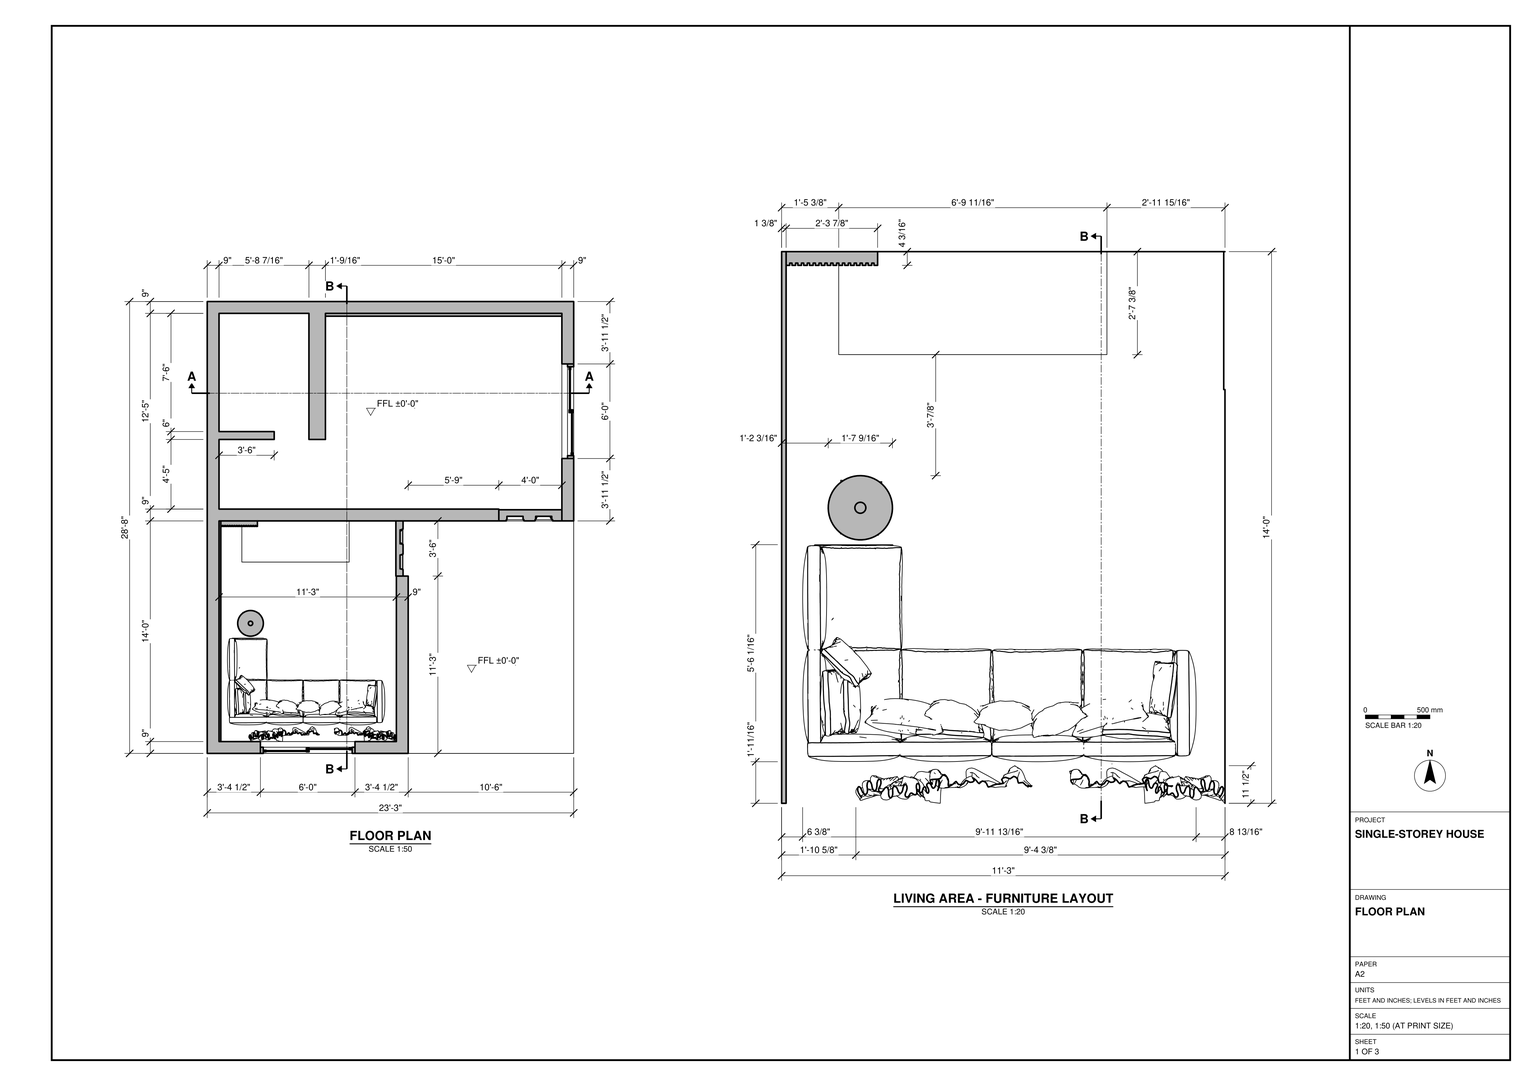
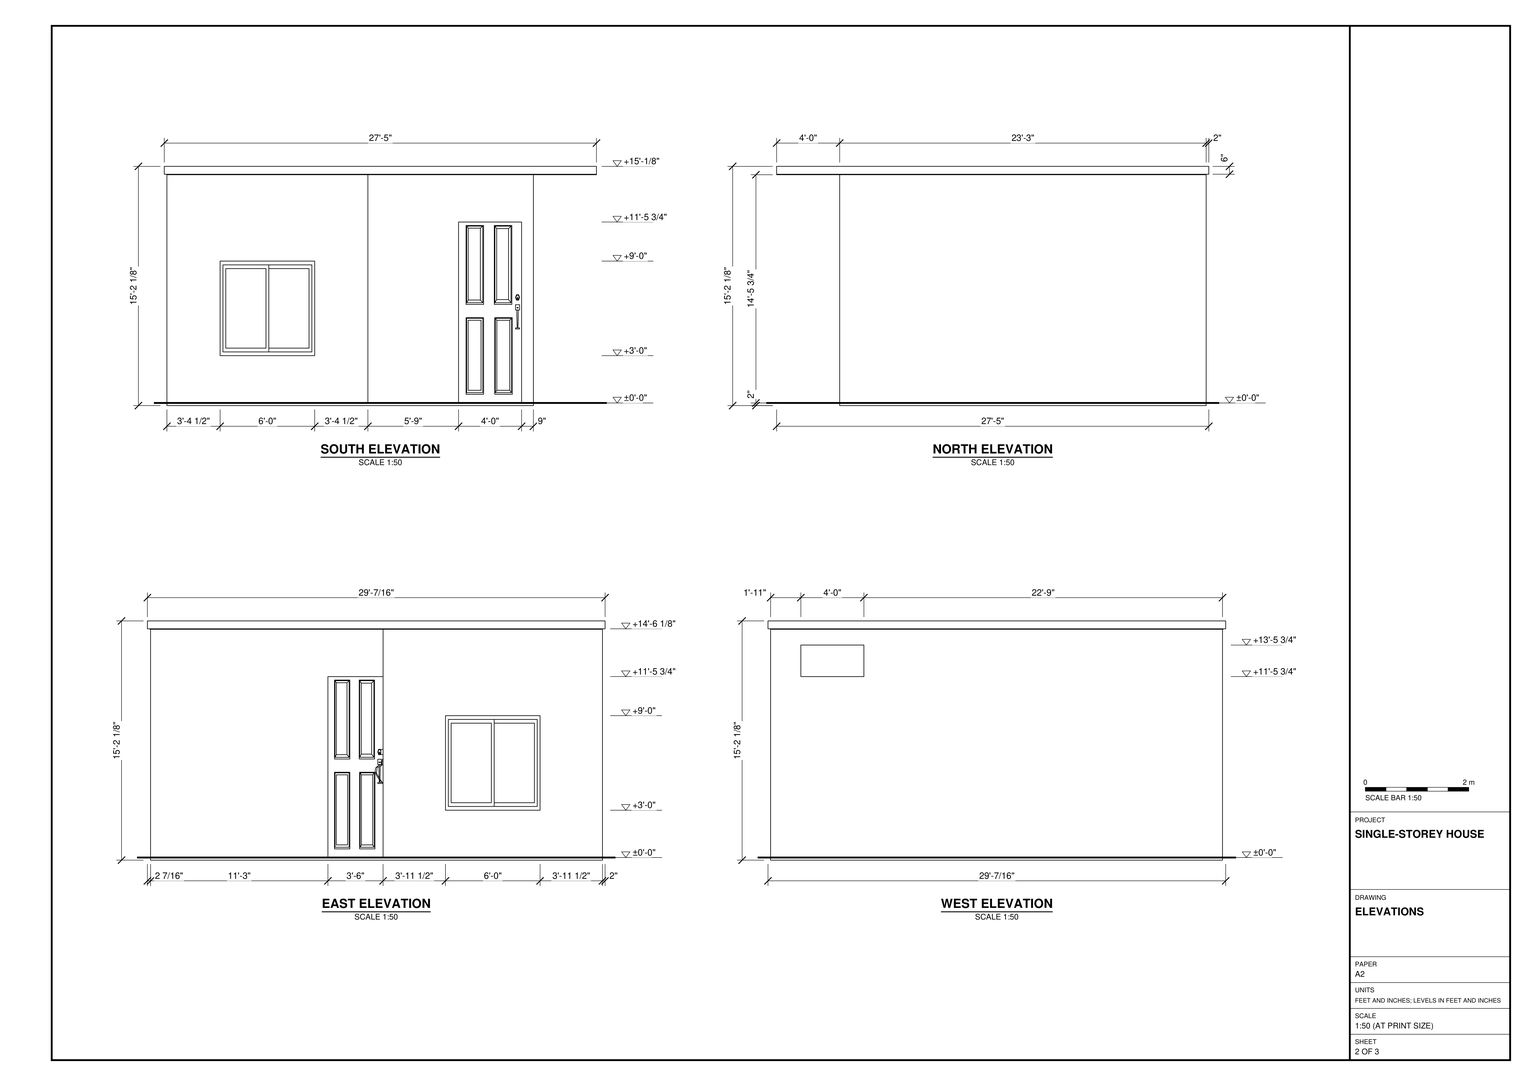
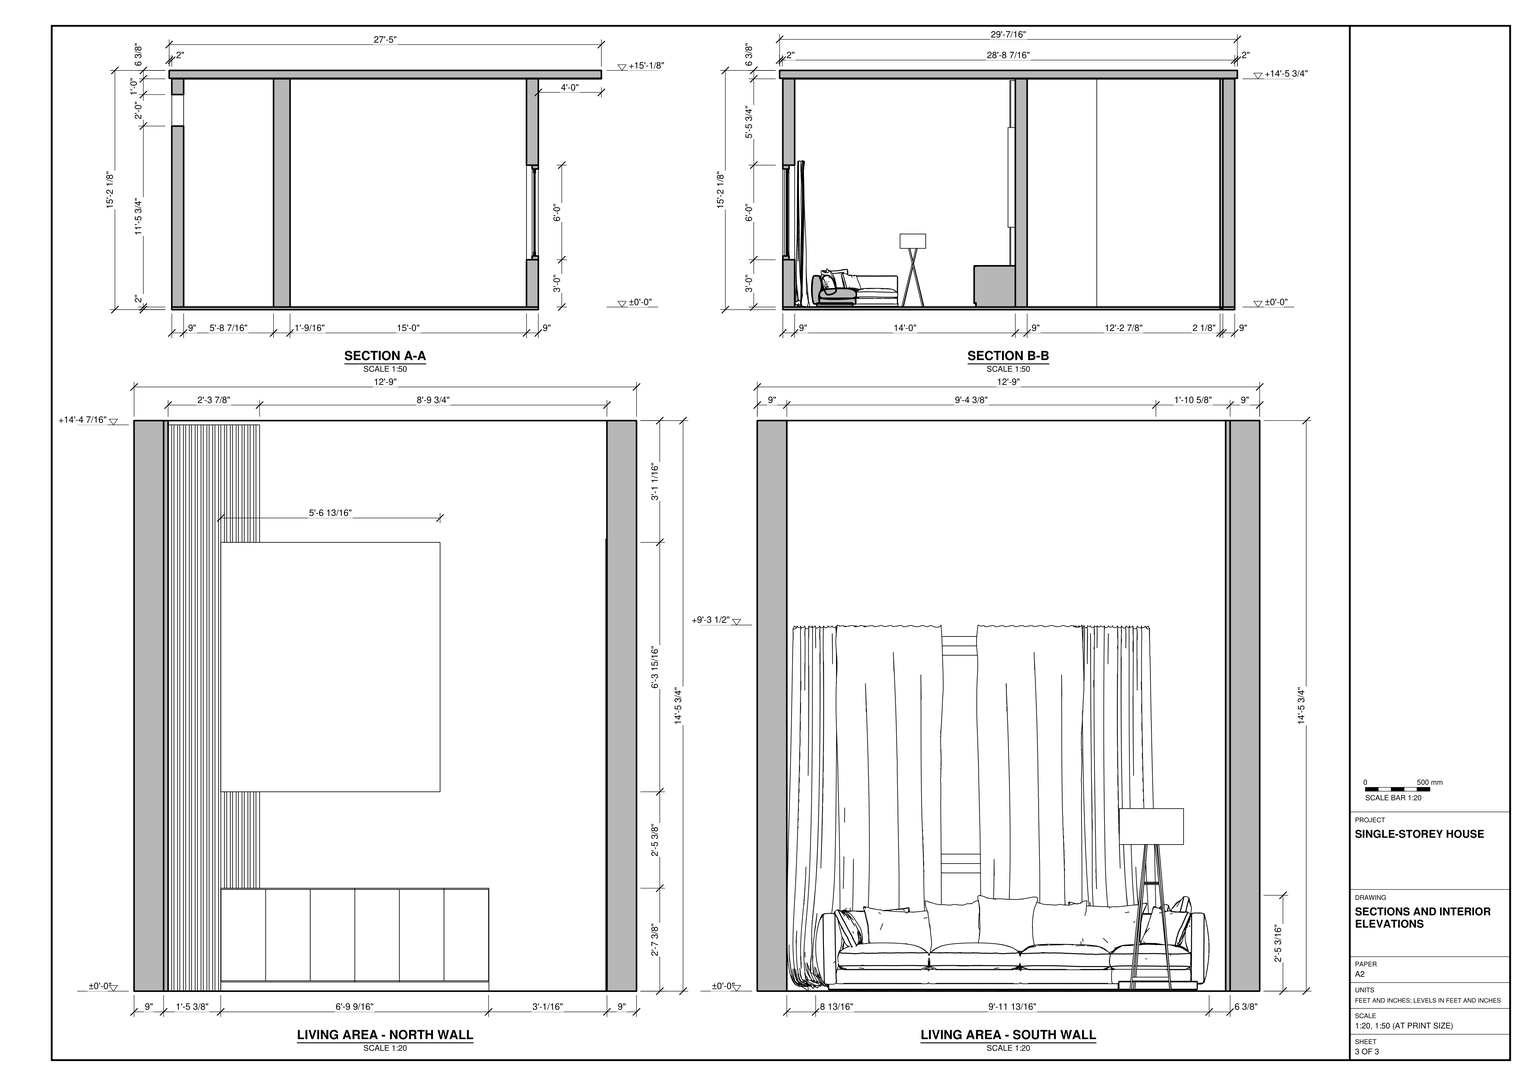
Build the single-storey house in SketchUp from task_files/diagram_01.pdf. Work in feet and inches. The overall model measures 27'-5" east to west, 29'-7/16" north to south and 15'-2 1/8" high. Set the finished floor level to ±0'-0" throughout.

Use the floor plan to lay out the wide northern part of the house and the narrower living area projecting south from its west end. Follow the wall thicknesses shown, including the 9" exterior walls and the different thicknesses of the internal partitions. Model the floor slab and the flat roof, using the sections to set their thicknesses and the roof overhangs. Fit the doors and window units in their respective wall openings, including the high opening in the west wall.

Use the enlarged furniture plan to place the sectional sofa in front of the south window, with its return along the west side. On the opposite wall, model the low cabinet, the rectangular panel above it and the narrow strip of vertical slats. Include the curtains, cushions and floor lamp in the positions shown. Decor and loose items may be any suitable library components.

Keep the walls, slabs and roof as separate groups or components, and group each furniture or joinery piece separately. Use components for repeated parts. Save one SketchUp model as output_files/single_storey_house_with_a_furnished_living_area.skp.

# SketchUp Ruby script. Lengths in inches.
U = 1.inch
M = Sketchup.active_model
def pt(a) = Geom::Point3d.new(a.map { |v| v * U })
def face(e, loops, mat)
  f = e.add_face(loops[0].map { |a| pt(a) })
  loops[1..].each { |l| e.add_face(l.map { |a| pt(a) }).erase! }
  f.material = f.back_material = mat if mat
  f
end
# faces: each face lists its corners as indices into pts; further lists are holes
def faces(e, pts, list, mat = nil) = list.each { |f| face(e, (f[0].is_a?(Array) ? f : [f]).map { |l| l.map { |i| pts[i] } }, mat) }
# xy, xz, yz: faces in a plane at the given z, y or x. An outline is a flat list of corners, or four numbers for a rectangle; further outlines are holes
def ring(l) = l.size == 4 ? [[l[0], l[1]], [l[2], l[1]], [l[2], l[3]], [l[0], l[3]]] : l.each_slice(2).to_a
def flat(e, list, mat, &to3) = list.each { |f| face(e, (f[0].is_a?(Array) ? f : [f]).map { |l| ring(l).map { |u, v| to3.(u, v) } }, mat) }
def xy(e, z, list, mat = nil) = flat(e, list, mat) { |x, y| [x, y, z] }
def xz(e, y, list, mat = nil) = flat(e, list, mat) { |x, z| [x, y, z] }
def yz(e, x, list, mat = nil) = flat(e, list, mat) { |y, z| [x, y, z] }
def lines(e, pts, list) = list.each { |a, b| e.add_line(pt(pts[a]), pt(pts[b])) }
# prism: a flat outline (further loops are holes) pulled along v
def prism(e, loops, v, mat = nil)
  f = face(e, loops, mat); d = Geom::Vector3d.new(v.map { |x| x * U })
  f.pushpull(f.normal.samedirection?(d) ? d.length : -d.length)
end
def box(e, o, s, mat = nil) = prism(e, [[o, [o[0] + s[0], o[1], o[2]], [o[0] + s[0], o[1] + s[1], o[2]], [o[0], o[1] + s[1], o[2]]]], [0, 0, s[2]], mat)
def at(x, y, z, deg = 0) = Geom::Transformation.translation(pt([x, y, z])) * Geom::Transformation.rotation(ORIGIN, Z_AXIS, deg.degrees)
def axes(o, x, y, z) = Geom::Transformation.new([*x, 0, *y, 0, *z, 0, *pt(o).to_a, 1])
def part(name) = M.definitions.add(name)
# library, detail: a bought-in or finely detailed component or shape, given as its bounding box
def library(name, o, s) = part(name).tap { |d| box(d.entities, o, s) }
def detail(e, o, s) = box(e.add_group.entities, o, s)
def put(e, d, t, mat = nil) = e.add_instance(d, t).tap { |i| i.material = mat if mat }
def group(e, t, mat = nil) = e.add_group.tap { |g| g.transformation = t; g.material = mat if mat }.entities
root = M.entities
M.materials.add("PDM_Wallquest_gs62702").color = [246, 247, 235]
M.materials.add("R16744_image1_8d25cb92-550f-4773-b1c3-d29ba8c2fed5_grande").color = [220, 220, 208]
M.materials.add("Stacy_Pants").color = [40, 58, 94]
M.materials.add("[Color_D02]").color = [255, 204, 50]
M.materials.add("[CoolGray4]").color = [225, 226, 230]
M.materials["[CoolGray4]"].alpha = 0.26
M.materials.add("[Wallpaper Thin Brown Stripes]").color = [175, 154, 113]
M.materials.add("[Wood_ Floor]").color = [165, 112, 65]
c1 = part("Wallquest_gs62702.skp")
box(c1.entities,[0,0,0],[39.37,39.37,39.37],"PDM_Wallquest_gs62702")
c2 = part("Wallpaper texure")
g1 = group(c2.entities,at(16.6875,16,0))
box(g1,[0,-0.5,0],[120,0.5,120],"R16744_image1_8d25cb92-550f-4773-b1c3-d29ba8c2fed5_grande")
c3 = library("cream sofa",[28.24,67.89,0],[128.61,101.73,111.49])
c4 = part("Window sash")
g2 = group(c4.entities,at(0.98,0,0))
prism(g2,[[[-0.98,0,0],[30.98,0,0],[30.98,0,45.6],[-0.98,0,45.6]],[[29.01,0,43.625],[29.01,0,1.97],[0.98,0,1.97],[0.98,0,43.625]]],[0,1.18,0])
g3 = group(c4.entities,at(1.97,0.59,1.97))
xz(g3,0,[[0,0,28.03,41.66]],"[CoolGray4]")
c5 = part("Sliding window")
put(c5.entities,c4,at(31.97,2.82,1.97))
put(c5.entities,c4,at(1.97,1.25,1.97))
g4 = group(c5.entities,at(0,0,0))
prism(g4,[[[65.9,4.72,0],[0,4.72,0],[0,4.72,49.53],[65.9,4.72,49.53]],[[1.97,4.72,47.5625],[1.97,4.72,1.97],[63.93,4.72,1.97],[63.93,4.72,47.5625]]],[0,-4.72,0])
c6 = part("doorknob_half")
xy(c6.entities,0,[[0,13.65,0,16.25,0.75,16.25,1.5,14.95,0.75,13.65]])
xy(c6.entities,0.25,[[0,0,1.5,0.5]])
xy(c6.entities,0.75,[[0,13.875,0.62,13.875,1.24,14.95,0.62,16.03,0,16.03,0,14.95,0.27,14.84,0.375,14.58,0.27,14.3125,0,14.2],[0,14.2,0.27,14.3125,0.375,14.58,0.27,14.84,0,14.95,0,14.56,0.0625,14.56,0.0625,14.31,0,14.31],[0,14.31,0.0625,14.56]])
xz(c6.entities,0,[[0,0,1.5,0.25]])
xz(c6.entities,0.5,[[0.25,0,1.5,0.25]])
xz(c6.entities,11.5,[[0,0,1.5,0.25]])
yz(c6.entities,0.5,[[8.47,1.63,7.4,2.45,7.67,1.97],[7.67,1.97,7.4,2.45,6.07,2.625]])
yz(c6.entities,1.5,[[0,0,0.5,0.25],[9,0,11.5,0,11.5,0.25,9,0.4]])
p = [[0.62,13.875,0.75],[0,13.875,0.75],[0,13.65,0],[0.75,13.65,0],[1.5,14.95,0],[1.24,14.95,0.75],
  [0.75,16.25,0],[0.62,16.03,0.75],[0,16.25,0],[0,16.03,0.75],[0,0.5,0.25],[0.25,0.5,0.25],
  [0.37,2.17,1.44],[0,2.17,1.44],[0.35,2.36,1.17],[1.5,11.5,0.25],[0,11.5,0.25],[0,10.1875,0.32],
  [0,9,0.4],[0.5,9,0.4],[1.5,9,0.4],[0.5,10.1875,0.32],[0,9.9375,1.32],[0.5,9.9375,1.32],
  [0.49,8.53,0.39],[0.5,8.47,1.63],[0.5,7.67,1.97],[0,8.47,1.63],[0.43,4.05,2.25],[0.45,4.92,2.17],
  [0,4.05,2.25],[0,7.4,2.45],[0.5,7.4,2.45],[0.5,6.07,2.625],[0,6.07,2.625]]
faces(c6.entities,p,[[0,1,2,3],[3,4,5,0],[5,4,6,7],[6,8,9,7],[10,11,12,13],[14,12,11],[15,16,17,18,19,20],[21,17,22,23],
  [24,25,26],[27,25,19,18],[25,24,19],[14,28,12],[28,14,29],[13,12,28,30],[31,32,25,27],[26,33,29],
  [30,28,33,34],[29,33,28],[34,33,32,31]])
c7 = part("Doorknob_HandleSet")
put(c7.entities,c6,at(1.5,0,0))
put(c7.entities,c6,axes([1.5,0,0],[-1,0,0],[0,1,0],[0,0,1]))
c8 = part("Untitled")
xy(c8.entities,0,[[0,0,107.75,8.5]])
xy(c8.entities,9.45,[[12.86,0,42.86,1],[61.86,0,91.86,1]],"[Wood_ Floor]")
xy(c8.entities,11.24,[[13.91,1,41.41,3.5],[62.91,1,90.41,3.5]],"[Wood_ Floor]")
xy(c8.entities,92.74,[[13.91,1,41.41,3.5],[62.91,1,90.41,3.5]],"[Wood_ Floor]")
xy(c8.entities,93.45,[[12.86,0,42.86,1],[61.86,0,91.86,1]],"[Wood_ Floor]")
xy(c8.entities,107.93,[[12.86,0,42.86,1],[61.11,0,91.11,1]],"[Wood_ Floor]")
xy(c8.entities,109.78,[[13.91,1,41.41,4],[62.16,1,89.66,4]],"[Wood_ Floor]")
xy(c8.entities,193.72,[[13.91,1,41.41,4],[62.16,1,89.66,4]],"[Wood_ Floor]")
xy(c8.entities,194.45,[[12.86,0,42.86,1],[61.11,0,91.11,1]],"[Wood_ Floor]")
xy(c8.entities,198.25,[[0,0,107.75,8.5]])
xz(c8.entities,0,[[[0,0,107.75,198.25],[12.86,9.45,12.86,93.45,42.86,93.45,42.86,9.45,61.86,9.45,61.86,93.45,91.86,93.45,91.86,9.45],[12.86,107.93,42.86,194.45],[61.11,107.93,91.11,194.45]]],"[Wood_ Floor]")
xz(c8.entities,1,[[[12.86,9.45,42.86,93.45],[13.91,11.24,41.41,92.74]],[[61.86,9.45,91.86,93.45],[62.91,11.24,90.41,92.74]],[[12.86,107.93,42.86,194.45],[13.91,109.78,41.41,193.72]],[[61.11,107.93,91.11,194.45],[62.16,109.78,89.66,193.72]]],"[Wood_ Floor]")
xz(c8.entities,3.5,[[[13.91,11.24,41.41,92.74],[16.47,13.85,38.47,90.6]],[[62.91,11.24,90.41,92.74],[65.47,13.85,87.47,90.6]],[16.47,13.85,38.47,90.6],[65.47,13.85,87.47,90.6]],"[Wood_ Floor]")
xz(c8.entities,4,[[[13.91,109.78,41.41,193.72],[16.57,112.78,37.32,191.53]],[[62.16,109.78,89.66,193.72],[65.2,113.3,85.45,191.05]],[16.57,112.78,37.32,191.53],[65.2,113.3,85.45,191.05]],"[Wood_ Floor]")
xz(c8.entities,8.5,[[0,0,107.75,198.25]],"[Wood_ Floor]")
yz(c8.entities,0,[[0,0,8.5,198.25]],"[Wood_ Floor]")
yz(c8.entities,12.86,[[0,9.45,1,93.45],[0,107.93,1,194.45]],"[Wood_ Floor]")
yz(c8.entities,13.91,[[1,11.24,3.5,92.74],[1,109.78,4,193.72]],"[Wood_ Floor]")
yz(c8.entities,41.41,[[1,11.24,3.5,92.74],[1,109.78,4,193.72]],"[Wood_ Floor]")
yz(c8.entities,42.86,[[0,9.45,1,93.45],[0,107.93,1,194.45]],"[Wood_ Floor]")
yz(c8.entities,61.11,[[0,107.93,1,194.45]],"[Wood_ Floor]")
yz(c8.entities,61.86,[[0,9.45,1,93.45]],"[Wood_ Floor]")
yz(c8.entities,62.16,[[1,109.78,4,193.72]],"[Wood_ Floor]")
yz(c8.entities,62.91,[[1,11.24,3.5,92.74]],"[Wood_ Floor]")
yz(c8.entities,89.66,[[1,109.78,4,193.72]],"[Wood_ Floor]")
yz(c8.entities,90.41,[[1,11.24,3.5,92.74]],"[Wood_ Floor]")
yz(c8.entities,91.11,[[0,107.93,1,194.45]],"[Wood_ Floor]")
yz(c8.entities,91.86,[[0,9.45,1,93.45]],"[Wood_ Floor]")
yz(c8.entities,107.75,[[0,0,8.5,198.25]],"[Wood_ Floor]")
p = [[62.91,1,11.24],[65.47,3.5,13.85],[65.47,3.5,90.6],[62.91,1,92.74],[90.41,1,11.24],[87.47,3.5,13.85],
  [90.41,1,92.74],[87.47,3.5,90.6],[16.57,4,112.78],[13.91,1,109.78],[41.41,1,109.78],[37.32,4,112.78],
  [16.57,4,191.53],[13.91,1,193.72],[41.41,1,193.72],[37.32,4,191.53],[65.2,4,113.3],[62.16,1,109.78],
  [89.66,1,109.78],[85.45,4,113.3],[65.2,4,191.05],[62.16,1,193.72],[89.66,1,193.72],[85.45,4,191.05]]
faces(c8.entities,p,[[0,1,2,3],[4,5,1,0],[5,4,6,7],[3,2,7,6],[8,9,10,11],[12,13,9,8],[11,10,14,15],[16,17,18,19],
  [17,16,20,21],[22,23,19,18],[21,20,23,22],[13,12,15,14]],"[Wood_ Floor]")
put(c8.entities,c7,axes([97.39,0,81.08],[2.31,0,0],[0,0,2.31],[0,-2.31,0]),"[Color_D02]")
xy(root,0,[[28.38,149.47,28.38,175.95,28.42,175.95,28.42,175.26,29.53,175.26,29.53,175.95,30.21,175.95,30.21,175.26,31.31,175.26,31.31,175.95,31.99,175.95,31.99,175.26,33.09,175.26,33.09,175.95,33.78,175.95,33.78,175.26,34.88,175.26,34.88,175.95,35.5625,175.95,35.5625,175.26,36.66,175.26,36.66,175.95,37.35,175.95,37.35,175.26,38.45,175.26,38.45,175.95,39.13,175.95,39.13,175.26,40.23,175.26,40.23,179.4375,110.06,179.4375,110.06,149.47],[12.37,175.26,12.37,179.4375,28.38,179.4375,28.38,175.95,27.74,175.95,27.74,175.26,26.64,175.26,26.64,175.95,25.96,175.95,25.96,175.26,24.86,175.26,24.86,175.95,24.17,175.95,24.17,175.26,23.07,175.26,23.07,175.95,22.39,175.95,22.39,175.26,21.29,175.26,21.29,175.95,20.6,175.95,20.6,175.26,19.5,175.26,19.5,175.95,18.82,175.95,18.82,175.26,17.72,175.26,17.72,175.95,17.04,175.95,17.04,175.26,15.94,175.26,15.94,175.95,15.25,175.95,15.25,175.26,14.15,175.26,14.15,175.95,13.47,175.95,13.47,175.26],[28.42,175.26,28.42,175.95,28.38,175.95,28.38,179.4375,40.23,179.4375,40.23,175.26,39.13,175.26,39.13,175.95,38.45,175.95,38.45,175.26,37.35,175.26,37.35,175.95,36.66,175.95,36.66,175.26,35.5625,175.26,35.5625,175.95,34.88,175.95,34.88,175.26,33.78,175.26,33.78,175.95,33.09,175.95,33.09,175.26,31.99,175.26,31.99,175.95,31.31,175.95,31.31,175.26,30.21,175.26,30.21,175.95,29.53,175.95,29.53,175.26]])
xy(root,2.79,[[28.38,148.08,110.06,149.47]])
xy(root,3.14,[[28.49,148.08,69.22,148.78],[69.22,148.08,82.8,148.78],[82.8,148.08,96.375,148.78],[96.375,148.08,109.95,148.78],[28.49,148.78,109.95,149.47]])
xy(root,3.16,[[28.49,148.08,42.07,148.78],[42.08,148.08,55.65,148.78],[55.66,148.08,69.22,148.78],[69.23,148.08,82.8,148.78],[82.81,148.08,96.375,148.78],
  [96.38,148.08,109.95,148.78],[28.49,148.78,69.22,149.47],[69.22,148.78,69.23,149.47],[69.23,148.78,109.95,149.47],[69.22,149.47,69.23,159.93]])
xy(root,30.98,[[28.49,148.08,42.07,148.78],[42.08,148.08,55.65,148.78],[55.66,148.08,69.22,148.78],[69.23,148.08,82.8,148.78],[82.81,148.08,96.375,148.78],
  [96.38,148.08,109.95,148.78],[28.49,148.78,69.22,149.47],[69.22,148.78,69.23,149.47],[69.23,148.78,109.95,149.47],[69.22,149.47,69.23,159.93]])
xy(root,31,[[28.49,148.08,69.22,148.78],[69.22,148.08,96.375,148.78],[96.375,148.08,109.95,148.78],[28.49,148.78,109.95,149.47]])
xy(root,31.36,[[28.38,148.08,110.06,179.4375]])
xy(root,60.72,[[28.38,173.86,95.1875,179.4375]])
xy(root,136.67,[[28.38,173.86,95.1875,179.4375]])
xy(root,172.46,[[12.37,175.26,13.47,175.95],[14.15,175.26,15.25,175.95],[15.94,175.26,17.04,175.95],[17.72,175.26,18.82,175.95],[19.5,175.26,20.6,175.95],
  [21.29,175.26,22.39,175.95],[23.07,175.26,24.17,175.95],[24.86,175.26,25.96,175.95],[26.64,175.26,27.74,175.95],[28.42,175.26,29.53,175.95],
  [30.21,175.26,31.31,175.95],[31.99,175.26,33.09,175.95],[33.78,175.26,34.88,175.95],[35.5625,175.26,36.66,175.95],[37.35,175.26,38.45,175.95],
  [39.13,175.26,40.23,175.95],[12.37,175.95,40.23,179.4375]])
xz(root,148.08,[[28.38,2.79,69.22,2.79,69.22,3.14,28.49,3.14,28.49,31,69.22,31,69.22,31.36,28.38,31.36],[69.22,2.79,82.8,3.14],[82.8,2.79,110.06,2.79,110.06,31.36,96.375,31.36,96.375,31,109.95,31,109.95,3.14,82.8,3.14],[28.49,3.16,42.07,30.98],[42.08,3.16,55.65,30.98],
  [55.66,3.16,69.22,30.98],[69.23,3.16,82.8,30.98],[82.81,3.16,96.375,30.98],[96.38,3.16,109.95,30.98],[69.22,31,96.375,31.36]])
xz(root,148.78,[[28.49,3.14,69.22,3.14,69.22,3.16,28.49,3.16,28.49,30.98,69.22,30.98,69.22,31,28.49,31],[69.22,3.14,82.8,3.16],[82.8,3.14,96.375,3.16],[96.375,3.14,109.95,3.14,109.95,31,96.375,31,96.375,30.98,109.95,30.98,109.95,3.16,96.375,3.16],[42.07,3.16,42.08,30.98],
  [55.65,3.16,55.66,30.98],[82.8,3.16,82.81,30.98],[96.375,3.16,96.38,30.98],[69.22,30.98,96.375,31]])
xz(root,149.47,[[28.38,0,110.06,2.79],[[28.49,3.14,109.95,31],[28.49,3.16,109.95,30.98]]])
xz(root,159.93,[[69.22,3.16,69.23,30.98]])
xz(root,173.86,[[28.38,60.72,95.1875,136.67]])
xz(root,175.26,[[12.37,0,13.47,172.46],[14.15,0,15.25,172.46],[15.94,0,17.04,172.46],[17.72,0,18.82,172.46],[19.5,0,20.6,172.46],
  [21.29,0,22.39,172.46],[23.07,0,24.17,172.46],[24.86,0,25.96,172.46],[26.64,0,27.74,172.46],[28.42,0,29.53,172.46],
  [30.21,0,31.31,172.46],[31.99,0,33.09,172.46],[33.78,0,34.88,172.46],[35.5625,0,36.66,172.46],[37.35,0,38.45,172.46],
  [39.13,0,40.23,172.46]])
xz(root,175.95,[[13.47,0,14.15,172.46],[15.25,0,15.94,172.46],[17.04,0,17.72,172.46],[18.82,0,19.5,172.46],[20.6,0,21.29,172.46],
  [22.39,0,23.07,172.46],[24.17,0,24.86,172.46],[25.96,0,26.64,172.46],[27.74,0,28.42,172.46],[29.53,0,30.21,172.46],
  [31.31,0,31.99,172.46],[33.09,0,33.78,172.46],[34.88,0,35.5625,172.46],[36.66,0,37.35,172.46],[38.45,0,39.13,172.46]],"Stacy_Pants")
xz(root,179.4375,[[12.37,0,12.37,172.46,40.23,172.46,40.23,136.67,28.38,136.67,28.38,60.72,40.23,60.72,40.23,31.36,28.38,31.36,28.38,0],[28.38,0,40.23,31.36],[40.23,0,110.06,31.36],[28.38,60.72,40.23,136.67],[40.23,60.72,95.1875,136.67]])
yz(root,12.37,[[175.26,0,179.4375,172.46]])
yz(root,13.47,[[175.26,0,175.95,172.46]])
yz(root,14.15,[[175.26,0,175.95,172.46]])
yz(root,15.25,[[175.26,0,175.95,172.46]])
yz(root,15.94,[[175.26,0,175.95,172.46]])
yz(root,17.04,[[175.26,0,175.95,172.46]])
yz(root,17.72,[[175.26,0,175.95,172.46]])
yz(root,18.82,[[175.26,0,175.95,172.46]])
yz(root,19.5,[[175.26,0,175.95,172.46]])
yz(root,20.6,[[175.26,0,175.95,172.46]])
yz(root,21.29,[[175.26,0,175.95,172.46]])
yz(root,22.39,[[175.26,0,175.95,172.46]])
yz(root,23.07,[[175.26,0,175.95,172.46]])
yz(root,24.17,[[175.26,0,175.95,172.46]])
yz(root,24.86,[[175.26,0,175.95,172.46]])
yz(root,25.96,[[175.26,0,175.95,172.46]])
yz(root,26.64,[[175.26,0,175.95,172.46]])
yz(root,27.74,[[175.26,0,175.95,172.46]])
yz(root,28.38,[[149.47,0,149.47,2.79,148.08,2.79,148.08,31.36,179.4375,31.36,179.4375,0],[173.86,60.72,179.4375,136.67]])
yz(root,28.42,[[175.26,0,175.95,172.46]])
yz(root,28.49,[[148.08,3.14,148.78,31],[148.78,3.14,149.47,31],[148.08,3.16,148.78,30.98],[148.78,3.16,149.47,30.98]])
yz(root,29.53,[[175.26,0,175.95,172.46]])
yz(root,30.21,[[175.26,0,175.95,172.46]])
yz(root,31.31,[[175.26,0,175.95,172.46]])
yz(root,31.99,[[175.26,0,175.95,172.46]])
yz(root,33.09,[[175.26,0,175.95,172.46]])
yz(root,33.78,[[175.26,0,175.95,172.46]])
yz(root,34.88,[[175.26,0,175.95,172.46]])
yz(root,35.5625,[[175.26,0,175.95,172.46]])
yz(root,36.66,[[175.26,0,175.95,172.46]])
yz(root,37.35,[[175.26,0,175.95,172.46]])
yz(root,38.45,[[175.26,0,175.95,172.46]])
yz(root,39.13,[[175.26,0,175.95,172.46]])
yz(root,40.23,[[175.26,0,175.95,172.46],[175.95,0,179.4375,172.46]])
yz(root,42.07,[[148.08,3.16,148.78,30.98]])
yz(root,42.08,[[148.08,3.16,148.78,30.98]])
yz(root,55.65,[[148.08,3.16,148.78,30.98]])
yz(root,55.66,[[148.08,3.16,148.78,30.98]])
yz(root,69.22,[[148.08,3.16,159.93,30.98]])
yz(root,69.23,[[148.08,3.16,159.93,30.98]])
yz(root,82.8,[[148.08,3.16,148.78,30.98]])
yz(root,82.81,[[148.08,3.16,148.78,30.98]])
yz(root,95.1875,[[173.86,60.72,179.4375,136.67]])
yz(root,96.375,[[148.08,3.16,148.78,30.98]])
yz(root,96.38,[[148.08,3.16,148.78,30.98]])
yz(root,109.95,[[148.08,3.14,148.78,31],[148.78,3.14,149.47,31],[148.08,3.16,148.78,30.98],[148.78,3.16,149.47,30.98]])
yz(root,110.06,[[149.47,0,179.4375,0,179.4375,31.36,148.08,31.36,148.08,2.79,149.47,2.79]])
yz(root,272,[[179.4375,137.75,188.4375,173.75]])
p = [[155,2.4375,0],[281,2.4375,0],[281,179.4375,0],[155,11.4375,0],[272,179.4375,0],[155,137.4375,137.75],
  [155,179.4375,137.75],[146,179.4375,137.75],[146,137.4375,137.75],[224,179.4375,137.75],[272,179.4375,137.75],[224,188.4375,137.75],
  [83,241.4375,137.75],[83,247.4375,137.75],[53,247.4375,137.75],[53,241.4375,137.75],[83,247.4375,173.75],[155,179.4375,173.75],
  [146,179.4375,173.75],[281,226.9375,36],[281,298.9375,36],[281,298.9375,108],[281,226.9375,108],[42.5,2.4375,36],
  [114.5,2.4375,36],[114.5,2.4375,108],[42.5,2.4375,108],[281,2.4375,-2],[281,2.4375,168.5625],[281,2.4375,175.5625]]
lines(root,p,[[0,1],[2,1],[0,3],[4,2],[5,6],[6,7],[5,8],[9,10],[9,11],[12,13],[14,15],[13,16],
  [17,18],[19,20],[20,21],[21,22],[22,19],[23,24],[24,25],[25,26],[26,23],[15,12],[27,1],[28,29],
  [1,28]])
put(root,c1,axes([92,337.4375,-0.875],[4.572,0,0],[0,-0.05462,0],[0,0,4.43545]))
put(root,c2,axes([54.75,202.8,0],[0,-1.4,0],[-2.73436,0,0],[0,0,1.44792]))
put(root,c3,at(174.25,181.05,0,180))
put(root,c5,axes([42.5,2.4375,36],[1.09255,0,0],[0,1,0],[0,0,1.45359]))
put(root,c5,axes([276.28,298.9375,36],[0,-1.09255,0],[1,0,0],[0,0,1.45359]))
put(root,c8,axes([224,179.4375,0],[0.44548,0,0],[0,1,0],[0,0,0.69483]))
put(root,c8,axes([151.1,137.4375,0],[0,0.38979,0],[-0.6439,0,0],[0,0,0.69483]))
g5 = group(root,at(2,-85.5625,0))
xy(g5,0,[[0,88,0,432,279,432,279,265,270,265,270,423,90,423,90,327,77.4375,327,77.4375,423,9,423,9,333,51,333,51,327,9,327,9,274,222,274,222,265,9,265,9,97,144,97,144,223,153,223,153,88]])
xy(g5,36,[[40.5,88,112.5,97],[270,312.5,279,384.5]])
xy(g5,108,[[40.5,88,112.5,97],[270,312.5,279,384.5]])
xy(g5,137.75,[[144,223,153,265],[51,327,77.4375,333],[0,360.99,9,408.99]])
xy(g5,137.75,[[222,265,270,274]],"PDM_Wallquest_gs62702")
xy(g5,161.75,[[0,360.99,9,408.99]])
xy(g5,173.75,[[0,88,153,88,153,265,144,265,144,97,9,97,9,265,222,265,222,274,9,274,9,327,51,327,51,333,9,333,9,423,77.4375,423,77.4375,333,51,333,51,327,90,327,90,423,270,423,270,265,279,265,279,432,0,432],[222,265,270,274]])
xz(g5,88,[[[0,0,153,173.75],[40.5,36,112.5,108]]])
xz(g5,97,[[[9,0,144,173.75],[40.5,36,112.5,108]]],"[Wallpaper Thin Brown Stripes]")
xz(g5,223,[[144,0,153,137.75]])
xz(g5,265,[[9,0,222,0,222,137.75,270,137.75,270,173.75,153,173.75,153,137.75,144,137.75,144,173.75,9,173.75],[270,0,279,173.75],[144,137.75,153,173.75]])
xz(g5,274,[[9,0,222,173.75],[222,137.75,270,173.75]],"PDM_Wallquest_gs62702")
xz(g5,312.5,[[270,36,279,108]])
xz(g5,327,[[9,0,51,173.75],[77.4375,0,90,0,90,173.75,81,173.75,81,137.75,77.4375,137.75],[51,137.75,81,173.75]],"PDM_Wallquest_gs62702")
xz(g5,333,[[9,0,51,173.75],[51,137.75,77.4375,173.75]])
xz(g5,360.99,[[0,137.75,9,161.75]])
xz(g5,384.5,[[270,36,279,108]])
xz(g5,408.99,[[0,137.75,9,161.75]])
xz(g5,423,[[9,0,77.4375,173.75]])
xz(g5,423,[[90,0,270,173.75]],"PDM_Wallquest_gs62702")
xz(g5,432,[[0,0,279,173.75]])
yz(g5,0,[[[88,0,432,173.75],[360.99,137.75,408.99,161.75]]])
yz(g5,9,[[97,0,265,173.75],[[333,0,423,173.75],[360.99,137.75,408.99,161.75]]])
yz(g5,9,[[274,0,327,173.75]],"PDM_Wallquest_gs62702")
yz(g5,40.5,[[88,36,97,108]])
yz(g5,51,[[327,0,333,137.75],[327,137.75,333,173.75]])
yz(g5,77.4375,[[327,0,327,137.75,333,137.75,333,173.75,423,173.75,423,0]])
yz(g5,90,[[327,0,423,173.75]],"PDM_Wallquest_gs62702")
yz(g5,112.5,[[88,36,97,108]])
yz(g5,144,[[97,0,223,173.75],[223,137.75,265,173.75]],"[Wallpaper Thin Brown Stripes]")
yz(g5,153,[[88,0,223,0,223,137.75,265,137.75,265,173.75,88,173.75]])
yz(g5,222,[[265,0,274,137.75]],"PDM_Wallquest_gs62702")
yz(g5,270,[[265,137.75,274,173.75]])
yz(g5,270,[[[265,0,265,137.75,274,137.75,274,173.75,423,173.75,423,0],[312.5,36,384.5,108]]],"PDM_Wallquest_gs62702")
yz(g5,279,[[[265,0,432,173.75],[312.5,36,384.5,108]]])
g6 = group(root,at(2,2.4375,-2))
box(g6,[0,0,0],[279,344,2])
g7 = group(root,at(2,2,173.75))
xy(g7,0,[[0,0,327,344.4375]])
xy(g7,0.375,[[-2,-2,0,346.4375],[0,-2,327,0],[0,0,327,344.4375],[0,344.4375,327,346.4375]])
xy(g7,6.375,[[-2,-2,327,346.4375]])
xz(g7,-2,[[-2,0.375,327,6.375]])
xz(g7,0,[[0,0,327,0.375]])
xz(g7,344.4375,[[0,0,327,0.375]])
xz(g7,346.4375,[[-2,0.375,327,6.375]])
yz(g7,-2,[[-2,0.375,346.4375,6.375]])
yz(g7,0,[[0,0,344.4375,0.375]])
yz(g7,327,[[0,0,344.4375,0.375],[-2,0.375,346.4375,6.375]])
